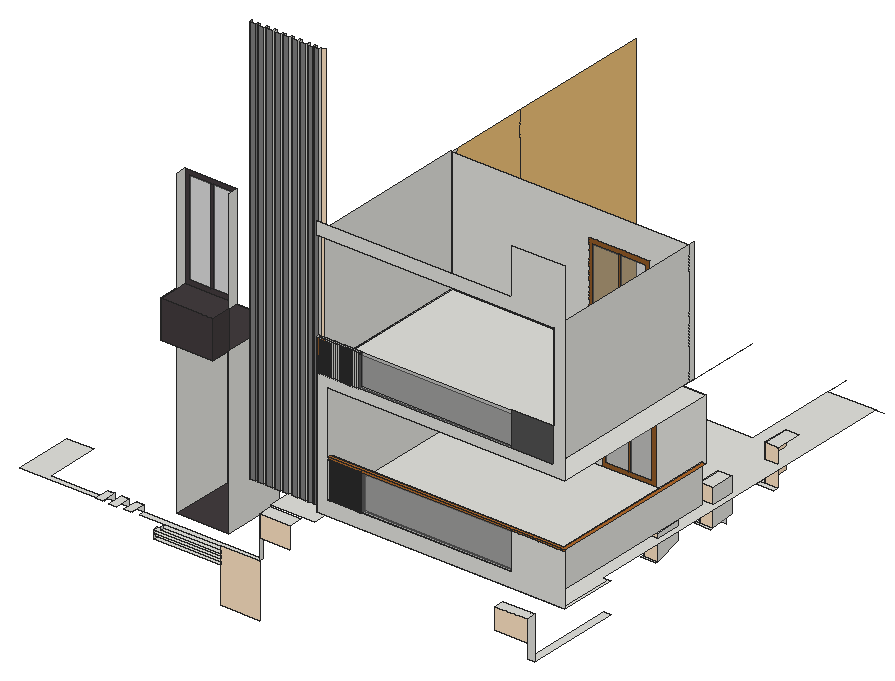
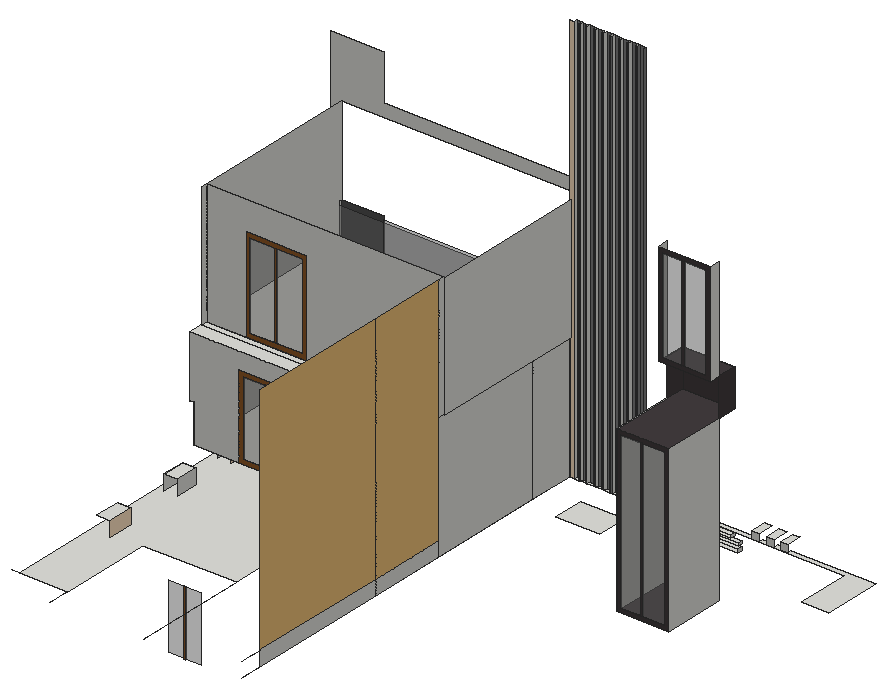
# SketchUp Ruby script. Lengths in inches.
U = 1.inch
M = Sketchup.active_model
def pt(a) = Geom::Point3d.new(a.map { |v| v * U })
def face(e, loops, mat)
  f = e.add_face(loops[0].map { |a| pt(a) })
  loops[1..].each { |l| e.add_face(l.map { |a| pt(a) }).erase! }
  f.material = f.back_material = mat if mat
  f
end
# faces: each face lists its corners as indices into pts; further lists are holes
def faces(e, pts, list, mat = nil) = list.each { |f| face(e, (f[0].is_a?(Array) ? f : [f]).map { |l| l.map { |i| pts[i] } }, mat) }
# xy, xz, yz: faces in a plane at the given z, y or x. An outline is a flat list of corners, or four numbers for a rectangle; further outlines are holes
def ring(l) = l.size == 4 ? [[l[0], l[1]], [l[2], l[1]], [l[2], l[3]], [l[0], l[3]]] : l.each_slice(2).to_a
def flat(e, list, mat, &to3) = list.each { |f| face(e, (f[0].is_a?(Array) ? f : [f]).map { |l| ring(l).map { |u, v| to3.(u, v) } }, mat) }
def xy(e, z, list, mat = nil) = flat(e, list, mat) { |x, y| [x, y, z] }
def xz(e, y, list, mat = nil) = flat(e, list, mat) { |x, z| [x, y, z] }
def yz(e, x, list, mat = nil) = flat(e, list, mat) { |y, z| [x, y, z] }
def lines(e, pts, list) = list.each { |a, b| e.add_line(pt(pts[a]), pt(pts[b])) }
# prism: a flat outline (further loops are holes) pulled along v
def prism(e, loops, v, mat = nil)
  f = face(e, loops, mat); d = Geom::Vector3d.new(v.map { |x| x * U })
  f.pushpull(f.normal.samedirection?(d) ? d.length : -d.length)
end
def box(e, o, s, mat = nil) = prism(e, [[o, [o[0] + s[0], o[1], o[2]], [o[0] + s[0], o[1] + s[1], o[2]], [o[0], o[1] + s[1], o[2]]]], [0, 0, s[2]], mat)
def at(x, y, z, deg = 0) = Geom::Transformation.translation(pt([x, y, z])) * Geom::Transformation.rotation(ORIGIN, Z_AXIS, deg.degrees)
def axes(o, x, y, z) = Geom::Transformation.new([*x, 0, *y, 0, *z, 0, *pt(o).to_a, 1])
def part(name) = M.definitions.add(name)
# library, detail: a bought-in or finely detailed component or shape, given as its bounding box
def library(name, o, s) = part(name).tap { |d| box(d.entities, o, s) }
def detail(e, o, s) = box(e.add_group.entities, o, s)
def put(e, d, t, mat = nil) = e.add_instance(d, t).tap { |i| i.material = mat if mat }
def group(e, t, mat = nil) = e.add_group.tap { |g| g.transformation = t; g.material = mat if mat }.entities
root = M.entities
M.materials.add("[0012_Bisque]").color = [255, 228, 196]
M.materials.add("[0133_Gray]").color = [128, 128, 128]
M.materials.add("[0135_DarkGray]").color = [81, 81, 81]
M.materials.add("[Asphalt New]").color = [67, 60, 62]
M.materials.add("[Translucent Glass Gray]").color = [128, 128, 128]
M.materials["[Translucent Glass Gray]"].alpha = 0.5
M.materials.add("[Wood Bamboo]").color = [177, 105, 43]
M.materials.add("[Wood Floor Parquet]").color = [145, 89, 39]
M.materials.add("[Wood OSB]").color = [240, 195, 122]
xy(root,46.08,[[99.93,136.77,144.79,190.64]],"[Asphalt New]")
xy(root,55.78,[[120.75,86.15,178.5,90.32]])
xy(root,58.72,[[120.75,86.15,178.5,90.32]])
xy(root,60.82,[[120.5,86.15,178.5,90.32]])
xy(root,63.13,[[120.5,86.15,178.5,90.32]])
xy(root,64.89,[[127.31,86.15,178.5,90.32]])
xy(root,67.33,[[127.31,86.15,178.5,90.32]])
xy(root,70.5625,[[5.25,86.15,78.43,86.15,78.43,90.09,84.2,90.09,84.2,86.15,89.84,86.15,89.84,90.32,28.64,90.32,28.64,136.77,5.25,136.77],[96.33,86.15,102.45,90.32],[109.08,86.15,211.95,90.32],[436.76,94.44,442.8125,176.35]])
xy(root,76.5625,[[78.43,76.52,84.2,90.09],[89.84,76.52,96.33,90.32],[102.45,76.52,109.08,90.32]])
xy(root,78.27,[[417.11,299.56,430.67,302],[417.11,302,419.11,322],[415.79,368,430.67,372.37],[415.79,372.37,419.11,395.12]])
xy(root,78.69,[[418.11,240,430.67,242.25],[418.11,242.25,419.11,264.5]])
xy(root,81.4,[[181.07,136.77,218.95,164.02]])
xy(root,96.9375,[[228.75,126.77,228.75,346.4375,313.66,346.4375,313.66,390.22,394.67,390.22,394.67,471.23,435.86,471.23,435.86,176.35,440.86,176.35,440.86,126.77],[440.86,126.77,443,176.35],[172.16,134.14,177.56,136.77],[179.41,134.14,184.81,136.77],[186.66,134.14,192.06,136.77],
  [193.91,134.14,199.31,136.77],[201.16,134.14,206.56,136.77],[208.41,134.14,213.81,136.77],[215.35,134.14,219.35,136.77],[220.74,134.14,224.75,136.77]])
xy(root,96.9375,[[164.91,134.14,170.31,136.77]],"[0133_Gray]")
xy(root,100.125,[[419.11,242.25,430.67,264.5]])
xy(root,107.1875,[[211.95,86.15,238.24,98.26],[415.52,86.15,442.8125,94.44]])
xy(root,109.68,[[238.59,126.77,239.95,129.8125],[239.95,126.77,241.32,129.8125],[241.32,126.77,242.02,129.8125],[242.02,126.77,243.5625,129.8125],[243.5625,126.77,244.14,129.8125],
  [244.14,126.77,245.6875,129.8125],[245.6875,126.77,246.27,129.8125],[246.27,126.77,247.8125,129.8125],[247.8125,126.77,248.39,129.8125],[248.39,126.77,249.9375,129.8125],
  [249.9375,126.77,250.52,129.8125],[250.52,126.77,252.0625,129.8125],[252.0625,126.77,252.64,129.8125],[252.64,126.77,254.1875,129.8125],[254.1875,126.77,254.77,129.8125],
  [254.77,126.77,256.3125,129.8125],[256.3125,126.77,256.89,129.8125],[256.89,126.77,258.4375,129.8125],[258.4375,126.77,259.02,129.8125],[259.02,126.77,260.5625,129.8125],
  [260.5625,126.77,261.14,129.8125],[261.14,126.77,262.6875,129.8125],[262.6875,126.77,263.27,129.8125],[263.27,126.77,264.8125,129.8125],[264.8125,126.77,265.39,129.8125],
  [265.39,126.77,266.38,129.8125],[266.38,126.77,266.7,129.8125],[238.59,129.8125,439.76,278.53],[419.11,302,430.67,322],[419.11,372.37,430.67,395.12]])
xy(root,140.87,[[238.59,126.77,239.95,129.8125],[239.95,126.77,241.32,129.8125],[241.32,126.77,242.02,129.8125],[242.02,126.77,243.5625,129.8125],[243.5625,126.77,244.14,129.8125],
  [244.14,126.77,245.6875,129.8125],[245.6875,126.77,246.27,129.8125],[246.27,126.77,247.8125,129.8125],[247.8125,126.77,248.39,129.8125],[248.39,126.77,249.9375,129.8125],
  [249.9375,126.77,250.52,129.8125],[250.52,126.77,252.0625,129.8125],[252.0625,126.77,252.64,129.8125],[252.64,126.77,254.1875,129.8125],[254.1875,126.77,254.77,129.8125],
  [254.77,126.77,256.3125,129.8125],[256.3125,126.77,256.89,129.8125],[256.89,126.77,258.4375,129.8125],[258.4375,126.77,259.02,129.8125],[259.02,126.77,260.5625,129.8125],
  [260.5625,126.77,261.14,129.8125],[261.14,126.77,262.6875,129.8125],[262.6875,126.77,263.27,129.8125],[263.27,126.77,264.8125,129.8125],[264.8125,126.77,265.39,129.8125],
  [265.39,126.77,266.38,129.8125],[266.38,126.77,266.7,129.8125],[266.7,126.77,267.84,129.8125]])
xy(root,142.87,[[238.59,126.77,443,126.77,443,278.53,439.76,278.53,439.76,129.8125,238.59,129.8125]],"[Wood Bamboo]")
xy(root,187.29,[[99.93,119.96,144.79,190.64]],"[Asphalt New]")
xy(root,195.98,[[238.59,126.77,443,278.53]])
xy(root,204.875,[[228.75,126.77,229.97,127.27],[229.97,126.77,231.29,127.27],[231.29,126.77,231.72,129.76],[231.72,126.77,233.04,127.39],[233.04,126.77,233.47,129.76],
  [233.47,126.77,234.79,127.46],[234.79,126.77,235.22,129.76],[235.22,126.77,236.54,127.64],[236.54,126.77,236.97,129.76],[236.97,126.77,238.29,127.46],
  [238.29,126.77,238.72,129.76],[238.72,126.77,240.04,127.64],[240.04,126.77,240.47,129.76],[240.47,126.77,241.79,127.33],[241.79,126.77,242.22,129.76],
  [242.22,126.77,243.54,127.27],[243.54,126.77,243.97,129.76],[243.97,126.77,245.29,127.27],[245.29,126.77,245.72,129.76],[245.72,126.77,247.04,127.27],
  [247.04,126.77,247.54,129.76],[247.54,126.77,248.85,127.27],[248.85,126.77,249.35,129.76],[249.35,126.77,250.67,127.27],[250.67,126.77,251.16,129.76],
  [251.16,126.77,252.48,127.27],[252.48,126.77,252.97,129.76],[252.97,126.77,254.29,127.27],[254.29,126.77,254.79,129.76],[254.79,126.77,256.1,127.27],
  [256.1,126.77,256.6,129.76],[256.6,126.77,257.92,127.27],[257.92,126.77,258.41,129.76],[258.41,126.77,259.73,127.27],[259.73,126.77,260.22,129.76],
  [260.22,126.77,261.54,127.27],[261.54,126.77,262.04,129.76],[262.04,126.77,263.35,127.27],[263.35,126.77,263.85,129.76],[263.85,126.77,265.17,127.27],
  [228.75,127.27,231.29,129.76],[242.22,127.27,243.54,129.76],[243.97,127.27,245.29,129.76],[245.72,127.27,247.04,129.76],[247.54,127.27,248.85,129.76],
  [249.35,127.27,250.67,129.76],[251.16,127.27,252.48,129.76],[252.97,127.27,254.29,129.76],[254.79,127.27,256.1,129.76],[256.6,127.27,257.92,129.76],
  [258.41,127.27,259.73,129.76],[260.22,127.27,261.54,129.76],[262.04,127.27,263.35,129.76],[240.47,127.33,241.79,129.76],[231.72,127.39,233.04,129.76],
  [233.47,127.46,234.79,129.76],[236.97,127.46,238.29,129.76],[235.22,127.64,236.54,129.76],[238.72,127.64,240.04,129.76],[228.75,129.76,433.38,272.95],
  [227.87,136.77,228.75,176.35],[227.87,176.35,228.75,272.95],[228.75,272.95,433.38,278.53]])
xy(root,219.85,[[99.93,119.96,144.79,146.21]],"[Asphalt New]")
xz(root,86.15,[[178.5,24.89,211.95,70.5625],[211.95,88.875,238.24,107.1875],[415.52,88.875,442.8125,107.1875]],"[0012_Bisque]")
xz(root,90.09,[[78.43,70.5625,84.2,76.5625]])
xz(root,90.32,[[89.84,70.5625,96.33,76.5625],[102.45,70.5625,109.08,76.5625]])
xz(root,94.44,[[436.76,70.5625,442.8125,107.1875]])
xz(root,119.96,[[99.93,187.29,144.79,219.85]],"[Asphalt New]")
xz(root,126.77,[[228.75,96.9375,443,96.9375,443,140.87,396.96,140.87,396.96,109.68,238.59,109.68,238.59,195.98,443,195.98,443,361.9375,396.96,361.9375,396.96,322.1875,228.75,322.1875,228.75,311.125,433.38,311.125,433.38,204.875,228.75,204.875]])
xz(root,126.77,[[396.96,204.875,433.38,235.06]],"[0135_DarkGray]")
xz(root,126.77,[[267.84,109.68,396.96,140.87],[265.17,204.875,396.96,232.0625]],"[Translucent Glass Gray]")
xz(root,126.77,[[239.95,109.68,241.32,140.87],[242.02,109.68,243.5625,140.87],[244.14,109.68,245.6875,140.87],[246.27,109.68,247.8125,140.87],[248.39,109.68,249.9375,140.87],
  [250.52,109.68,252.0625,140.87],[252.64,109.68,254.1875,140.87],[254.77,109.68,256.3125,140.87],[256.89,109.68,258.4375,140.87],[259.02,109.68,260.5625,140.87],
  [261.14,109.68,262.6875,140.87],[263.27,109.68,264.8125,140.87],[265.39,109.68,266.38,140.87],[266.7,109.68,267.84,140.87],[238.59,140.87,443,142.87],
  [231.29,204.875,231.72,232.0625],[233.04,204.875,233.47,232.0625],[234.79,204.875,235.22,232.0625],[236.54,204.875,236.97,232.0625],[238.29,204.875,238.72,232.0625],
  [240.04,204.875,240.47,232.0625],[241.79,204.875,242.22,232.0625],[243.54,204.875,243.97,232.0625],[245.29,204.875,245.72,232.0625],[247.04,204.875,247.54,232.0625],
  [248.85,204.875,249.35,232.0625],[250.67,204.875,251.16,232.0625],[252.48,204.875,252.97,232.0625],[254.29,204.875,254.79,232.0625],[256.1,204.875,256.6,232.0625],
  [257.92,204.875,258.41,232.0625],[259.73,204.875,260.22,232.0625],[261.54,204.875,262.04,232.0625],[263.35,204.875,263.85,232.0625]],"[Wood Bamboo]")
xz(root,127.27,[[228.75,204.875,231.29,232.0625],[242.22,204.875,243.54,232.0625],[243.97,204.875,245.29,232.0625],[245.72,204.875,247.04,232.0625],[247.54,204.875,248.85,232.0625],
  [249.35,204.875,250.67,232.0625],[251.16,204.875,252.48,232.0625],[252.97,204.875,254.29,232.0625],[254.79,204.875,256.1,232.0625],[256.6,204.875,257.92,232.0625],
  [258.41,204.875,259.73,232.0625],[260.22,204.875,261.54,232.0625],[262.04,204.875,263.35,232.0625],[263.85,204.875,265.17,232.0625]],"[Wood Bamboo]")
xz(root,127.33,[[240.47,204.875,241.79,232.0625]],"[Wood Bamboo]")
xz(root,127.39,[[231.72,204.875,233.04,232.0625]],"[Wood Bamboo]")
xz(root,127.46,[[233.47,204.875,234.79,232.0625],[236.97,204.875,238.29,232.0625]],"[Wood Bamboo]")
xz(root,127.64,[[235.22,204.875,236.54,232.0625],[238.72,204.875,240.04,232.0625]],"[Wood Bamboo]")
xz(root,129.76,[[228.75,204.875,231.29,232.0625],[231.72,204.875,233.04,232.0625],[233.47,204.875,234.79,232.0625],[235.22,204.875,236.54,232.0625],[236.97,204.875,238.29,232.0625],
  [238.72,204.875,240.04,232.0625],[240.47,204.875,241.79,232.0625],[242.22,204.875,243.54,232.0625],[243.97,204.875,245.29,232.0625],[245.72,204.875,247.04,232.0625],
  [247.54,204.875,248.85,232.0625],[249.35,204.875,250.67,232.0625],[251.16,204.875,252.48,232.0625],[252.97,204.875,254.29,232.0625],[254.79,204.875,256.1,232.0625],
  [256.6,204.875,257.92,232.0625],[258.41,204.875,259.73,232.0625],[260.22,204.875,261.54,232.0625],[262.04,204.875,263.35,232.0625],[263.85,204.875,265.17,232.0625]])
xz(root,129.76,[[265.17,204.875,433.38,232.0625]],"[Translucent Glass Gray]")
xz(root,129.8125,[[239.95,109.68,241.32,140.87],[242.02,109.68,243.5625,140.87],[244.14,109.68,245.6875,140.87],[246.27,109.68,247.8125,140.87],[248.39,109.68,249.9375,140.87],
  [250.52,109.68,252.0625,140.87],[252.64,109.68,254.1875,140.87],[254.77,109.68,256.3125,140.87],[256.89,109.68,258.4375,140.87],[259.02,109.68,260.5625,140.87],
  [261.14,109.68,262.6875,140.87],[263.27,109.68,264.8125,140.87],[265.39,109.68,266.38,140.87],[266.7,109.68,267.84,140.87],[396.96,109.68,439.76,140.87],
  [238.59,140.87,439.76,142.87]])
xz(root,129.8125,[[267.84,109.68,396.96,140.87]],"[Translucent Glass Gray]")
xz(root,134.14,[[164.91,96.9375,170.31,450.1],[172.16,96.9375,177.56,450.1],[179.41,96.9375,184.81,450.1],[186.66,96.9375,192.06,450.1],[193.91,96.9375,199.31,450.1],
  [201.16,96.9375,206.56,450.1],[208.41,96.9375,213.81,450.1],[215.35,96.9375,219.35,450.1],[220.74,96.9375,224.75,450.1]],"[0133_Gray]")
xz(root,136.77,[[224.75,96.9375,228.75,96.9375,228.75,204.875,227.87,204.875,227.87,311.125,228.75,311.125,228.75,450.1,224.75,450.1]],"[0012_Bisque]")
xz(root,136.77,[[170.31,96.9375,172.16,450.1],[177.56,96.9375,179.41,450.1],[184.81,96.9375,186.66,450.1],[192.06,96.9375,193.91,450.1],[199.31,96.9375,201.16,450.1],
  [206.56,96.9375,208.41,450.1],[213.81,96.9375,215.35,450.1],[219.35,96.9375,220.74,450.1]],"[0133_Gray]")
xz(root,146.21,[[[99.93,219.85,144.79,308.65],[103.5,223.42,141.23,305.09]],[122.36,223.42,124.41,305.09]],"[Asphalt New]")
xz(root,146.21,[[103.5,223.42,122.36,305.09],[124.41,223.42,141.23,305.09]],"[Translucent Glass Gray]")
xz(root,190.64,[[[99.93,46.08,144.79,187.29],[103.42,49.57,141.31,183.8]],[122.36,49.57,124.71,183.8]],"[Asphalt New]")
xz(root,190.64,[[103.42,49.57,122.36,183.8],[124.71,49.57,141.31,183.8]],"[Translucent Glass Gray]")
xz(root,242.25,[[419.11,78.69,430.67,100.125]],"[0012_Bisque]")
xz(root,272.95,[[227.87,204.875,228.75,311.125],[228.75,204.875,346.47,204.875,346.47,286.5625,399.66,286.5625,399.66,204.875,433.38,204.875,433.38,311.125,228.75,311.125]])
xz(root,272.95,[[350.54,208.94,373.07,282.49],[374.78,208.94,395.59,282.49]],"[Translucent Glass Gray]")
xz(root,272.95,[[[346.47,204.875,399.66,286.5625],[350.54,208.94,395.59,282.49]],[373.07,208.94,374.78,282.49]],"[Wood Floor Parquet]")
xz(root,278.53,[[238.59,109.68,353.15,109.68,353.15,181.12,400.72,181.12,400.72,109.68,439.76,109.68,439.76,142.87,443,142.87,443,195.98,238.59,195.98]])
xz(root,278.53,[[356.72,113.25,376.93,177.56],[378.64,113.25,397.15,177.56]],"[Translucent Glass Gray]")
xz(root,278.53,[[[353.15,109.68,400.72,181.12],[356.72,113.25,397.15,177.56]],[376.93,113.25,378.64,177.56]],"[Wood Floor Parquet]")
xz(root,302,[[419.11,78.27,430.67,109.68]],"[0012_Bisque]")
xz(root,372.37,[[419.11,78.27,430.67,109.68]],"[0012_Bisque]")
xz(root,390.22,[[343.67,21.55,357.77,78],[359.1875,21.55,371.875,78]],"[Translucent Glass Gray]")
xz(root,390.22,[[357.77,21.55,359.1875,78]],"[Wood Floor Parquet]")
yz(root,99.93,[[136.77,46.08,190.64,187.29],[136.77,219.85,146.21,308.65]])
yz(root,99.93,[[119.96,187.29,136.77,219.85]],"[Asphalt New]")
yz(root,120.5,[[86.15,60.82,90.32,63.13]])
yz(root,120.75,[[86.15,55.78,90.32,58.72]])
yz(root,127.31,[[86.15,64.89,90.32,67.33]])
yz(root,144.79,[[136.77,46.08,190.64,187.29],[136.77,219.85,146.21,308.65]])
yz(root,144.79,[[119.96,187.29,136.77,219.85]],"[Asphalt New]")
yz(root,164.91,[[134.14,96.9375,136.77,450.1]],"[0133_Gray]")
yz(root,170.31,[[134.14,96.9375,136.77,450.1]],"[0133_Gray]")
yz(root,172.16,[[134.14,96.9375,136.77,450.1]])
yz(root,177.56,[[134.14,96.9375,136.77,450.1]])
yz(root,178.5,[[86.15,55.78,90.32,58.72],[86.15,60.82,90.32,63.13],[86.15,64.89,90.32,67.33]])
yz(root,179.41,[[134.14,96.9375,136.77,450.1]])
yz(root,184.81,[[134.14,96.9375,136.77,450.1]])
yz(root,186.66,[[134.14,96.9375,136.77,450.1]])
yz(root,192.06,[[134.14,96.9375,136.77,450.1]])
yz(root,193.91,[[134.14,96.9375,136.77,450.1]])
yz(root,199.31,[[134.14,96.9375,136.77,450.1]])
yz(root,201.16,[[134.14,96.9375,136.77,450.1]])
yz(root,206.56,[[134.14,96.9375,136.77,450.1]])
yz(root,208.41,[[134.14,96.9375,136.77,450.1]])
yz(root,211.95,[[86.15,70.5625,90.32,107.1875]])
yz(root,213.81,[[134.14,96.9375,136.77,450.1]])
yz(root,215.35,[[134.14,96.9375,136.77,450.1]])
yz(root,219.35,[[134.14,96.9375,136.77,450.1]])
yz(root,220.74,[[134.14,96.9375,136.77,450.1]])
yz(root,224.75,[[134.14,96.9375,136.77,450.1]])
yz(root,227.87,[[136.77,204.875,272.95,311.125]])
yz(root,228.75,[[126.77,96.9375,136.77,204.875],[136.77,96.9375,176.35,204.875],[176.35,96.9375,278.53,204.875],[278.53,96.9375,346.4375,109.68],[346.4375,96.9375,471.23,109.68],
  [127.27,204.875,129.76,232.0625],[272.95,204.875,278.53,311.125]])
yz(root,228.75,[[278.53,109.68,346.4375,311.125],[346.4375,109.68,471.23,311.125]],"[Wood OSB]")
yz(root,229.97,[[126.78,204.87,126.78,204.875,127.27,204.875],[126.78,204.875,126.28,232.05,126.77,232.0625,127.27,204.875]],"[Wood Floor Parquet]")
yz(root,230.39,[[126.78,204.87,127.27,204.875,126.77,232.0625,126.28,232.05]],"[Wood Floor Parquet]")
yz(root,231.29,[[126.77,204.875,127.27,232.0625],[127.27,204.875,129.76,232.0625]])
yz(root,231.72,[[126.77,204.875,127.39,232.0625],[127.39,204.875,129.76,232.0625]])
yz(root,233.04,[[126.77,204.875,127.39,232.0625],[127.39,204.875,129.76,232.0625]])
yz(root,233.47,[[127.46,204.875,129.76,232.0625]])
yz(root,233.47,[[126.77,204.875,127.46,232.0625]],"[Wood Bamboo]")
yz(root,234.79,[[126.77,204.875,127.46,232.0625],[127.46,204.875,129.76,232.0625]])
yz(root,235.22,[[127.64,204.875,129.76,232.0625]])
yz(root,235.22,[[126.77,204.875,127.64,232.0625]],"[Wood Bamboo]")
yz(root,236.54,[[126.77,204.875,127.64,232.0625],[127.64,204.875,129.76,232.0625]])
yz(root,236.97,[[126.77,204.875,127.46,232.0625],[127.46,204.875,129.76,232.0625]])
yz(root,238.29,[[126.77,204.875,127.46,232.0625],[127.46,204.875,129.76,232.0625]])
yz(root,238.59,[[126.77,109.68,278.53,109.68,278.53,195.98,126.77,195.98,126.77,142.87,129.8125,142.87,129.8125,140.87,126.77,140.87]])
yz(root,238.72,[[126.77,204.875,127.64,232.0625],[127.64,204.875,129.76,232.0625]])
yz(root,239.95,[[126.77,109.68,129.8125,140.87]])
yz(root,240.04,[[126.77,204.875,127.64,232.0625],[127.64,204.875,129.76,232.0625]])
yz(root,240.47,[[126.77,204.875,127.33,232.0625],[127.33,204.875,129.76,232.0625]])
yz(root,241.32,[[126.77,109.68,129.8125,140.87]])
yz(root,241.79,[[126.77,204.875,127.33,232.0625],[127.33,204.875,129.76,232.0625]])
yz(root,242.02,[[126.77,109.68,129.8125,140.87]])
yz(root,242.22,[[126.77,204.875,127.27,232.0625],[127.27,204.875,129.76,232.0625]])
yz(root,243.54,[[126.77,204.875,127.27,232.0625],[127.27,204.875,129.76,232.0625]])
yz(root,243.5625,[[126.77,109.68,129.8125,140.87]])
yz(root,243.97,[[126.77,204.875,127.27,232.0625],[127.27,204.875,129.76,232.0625]])
yz(root,244.14,[[126.77,109.68,129.8125,140.87]])
yz(root,245.29,[[126.77,204.875,127.27,232.0625],[127.27,204.875,129.76,232.0625]])
yz(root,245.6875,[[126.77,109.68,129.8125,140.87]])
yz(root,245.72,[[126.77,204.875,127.27,232.0625],[127.27,204.875,129.76,232.0625]])
yz(root,246.27,[[126.77,109.68,129.8125,140.87]])
yz(root,247.04,[[126.77,204.875,127.27,232.0625],[127.27,204.875,129.76,232.0625]])
yz(root,247.54,[[126.77,204.875,127.27,232.0625],[127.27,204.875,129.76,232.0625]])
yz(root,247.8125,[[126.77,109.68,129.8125,140.87]])
yz(root,248.39,[[126.77,109.68,129.8125,140.87]])
yz(root,248.85,[[126.77,204.875,127.27,232.0625],[127.27,204.875,129.76,232.0625]])
yz(root,249.35,[[126.77,204.875,127.27,232.0625],[127.27,204.875,129.76,232.0625]])
yz(root,249.9375,[[126.77,109.68,129.8125,140.87]])
yz(root,250.52,[[126.77,109.68,129.8125,140.87]])
yz(root,250.67,[[126.77,204.875,127.27,232.0625],[127.27,204.875,129.76,232.0625]])
yz(root,251.16,[[126.77,204.875,127.27,232.0625],[127.27,204.875,129.76,232.0625]])
yz(root,252.0625,[[126.77,109.68,129.8125,140.87]])
yz(root,252.48,[[126.77,204.875,127.27,232.0625],[127.27,204.875,129.76,232.0625]])
yz(root,252.64,[[126.77,109.68,129.8125,140.87]])
yz(root,252.97,[[126.77,204.875,127.27,232.0625],[127.27,204.875,129.76,232.0625]])
yz(root,254.1875,[[126.77,109.68,129.8125,140.87]])
yz(root,254.29,[[126.77,204.875,127.27,232.0625],[127.27,204.875,129.76,232.0625]])
yz(root,254.77,[[126.77,109.68,129.8125,140.87]])
yz(root,254.79,[[126.77,204.875,127.27,232.0625],[127.27,204.875,129.76,232.0625]])
yz(root,256.1,[[126.77,204.875,127.27,232.0625],[127.27,204.875,129.76,232.0625]])
yz(root,256.3125,[[126.77,109.68,129.8125,140.87]])
yz(root,256.6,[[126.77,204.875,127.27,232.0625],[127.27,204.875,129.76,232.0625]])
yz(root,256.89,[[126.77,109.68,129.8125,140.87]])
yz(root,257.92,[[126.77,204.875,127.27,232.0625],[127.27,204.875,129.76,232.0625]])
yz(root,258.41,[[126.77,204.875,127.27,232.0625],[127.27,204.875,129.76,232.0625]])
yz(root,258.4375,[[126.77,109.68,129.8125,140.87]])
yz(root,259.02,[[126.77,109.68,129.8125,140.87]])
yz(root,259.73,[[126.77,204.875,127.27,232.0625],[127.27,204.875,129.76,232.0625]])
yz(root,260.22,[[126.77,204.875,127.27,232.0625],[127.27,204.875,129.76,232.0625]])
yz(root,260.5625,[[126.77,109.68,129.8125,140.87]])
yz(root,261.14,[[126.77,109.68,129.8125,140.87]])
yz(root,261.54,[[126.77,204.875,127.27,232.0625],[127.27,204.875,129.76,232.0625]])
yz(root,262.04,[[126.77,204.875,127.27,232.0625],[127.27,204.875,129.76,232.0625]])
yz(root,262.6875,[[126.77,109.68,129.8125,140.87]])
yz(root,263.27,[[126.77,109.68,129.8125,140.87]])
yz(root,263.35,[[126.77,204.875,127.27,232.0625],[127.27,204.875,129.76,232.0625]])
yz(root,263.85,[[126.77,204.875,127.27,232.0625],[127.27,204.875,129.76,232.0625]])
yz(root,264.8125,[[126.77,109.68,129.8125,140.87]])
yz(root,265.17,[[126.77,204.875,127.27,232.0625]])
yz(root,265.39,[[126.77,109.68,129.8125,140.87]])
yz(root,266.38,[[126.77,109.68,129.8125,140.87]])
yz(root,266.7,[[126.77,109.68,129.8125,140.87]])
yz(root,419.11,[[302,78.27,322,109.68]])
yz(root,419.11,[[372.37,78.27,395.12,109.68],[242.25,78.69,264.5,100.125]],"[0012_Bisque]")
yz(root,430.67,[[302,78.27,322,80.77,322,109.68,302,109.68],[242.25,78.69,242.37,78.73,242.37,89.75,242.25,89.75],[242.37,78.73,264.5,84.8125,264.5,100.125,242.25,100.125,242.25,89.75,242.37,89.75]])
yz(root,433.38,[[129.76,204.875,129.76,235.06,126.77,235.06,126.77,311.125,272.95,311.125,272.95,204.875],[272.95,204.875,278.53,311.125]])
yz(root,439.76,[[129.8125,109.68,278.53,142.87]])
p = [[229.97,126.28,232.05],[229.97,126.78,204.875],[229.97,126.78,204.87],[230.39,126.78,204.87],[230.39,126.28,232.05],[229.97,127.27,204.875],
  [230.39,127.27,204.875],[229.97,126.77,232.0625],[230.39,126.77,232.0625],[313.66,390.22,96.9375],[313.66,471.23,96.9375],[394.67,471.23,96.9375],
  [394.67,490.875,96.9375],[313.66,490.875,96.9375],[435.86,471.23,96.9375],[443,471.23,96.9375],[228.75,490.875,96.9375],[228.75,471.23,96.9375],
  [228.75,471.23,109.68],[228.75,490.875,109.68]]
faces(root,p,[[0,1,2,3,4],[5,6,3,2],[5,7,8,6]],"[Wood Floor Parquet]")
lines(root,p,[[9,10],[11,12],[10,13],[14,15],[16,17],[18,19]])
